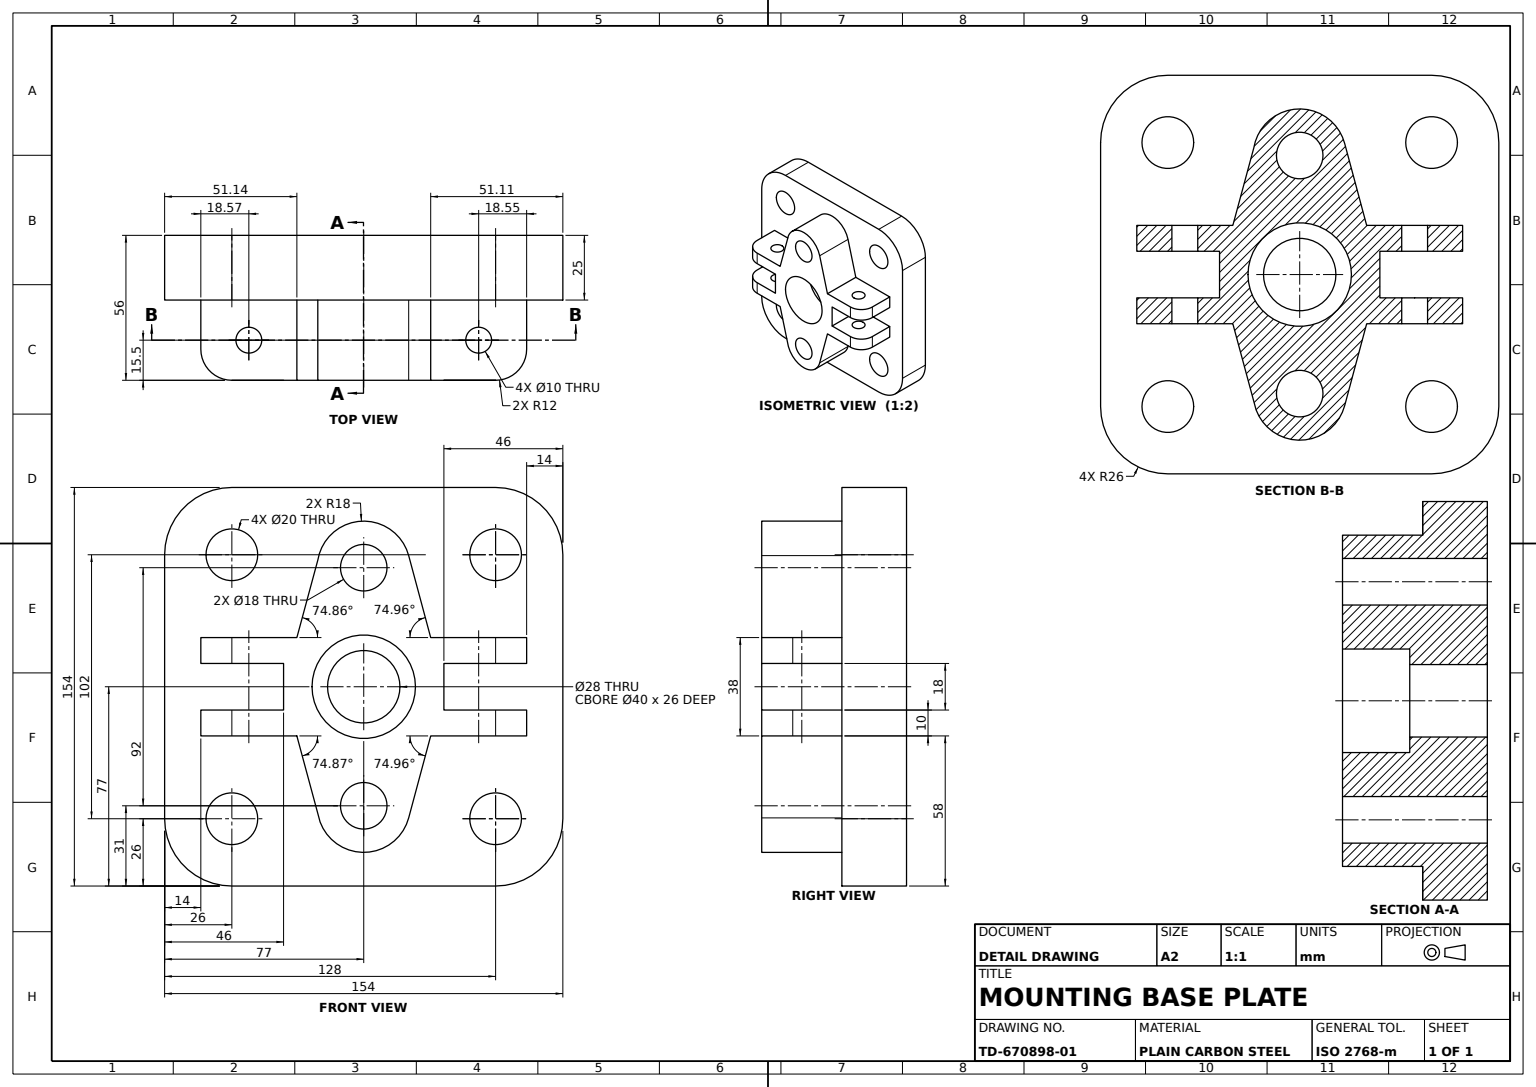
solid
v1 (97,77,56)
v2 (57,77,56)
e1 v1 v2 CIRCLE(AX(P(77,77,56),D(0,0,1),D(1,0,0)),20)
e2 v2 v1 CIRCLE(AX(P(77,77,56),D(0,0,1),D(1,0,0)),20)
v3 (86,31,56)
v4 (68,31,56)
e3 v3 v4 CIRCLE(AX(P(77,31,56),D(0,0,1),D(1,0,0)),9)
e4 v4 v3 CIRCLE(AX(P(77,31,56),D(0,0,1),D(1,0,0)),9)
v5 (108,86,56)
v6 (108,68,56)
e5 v5 v6 LINE
v7 (128,86,56)
e6 v5 v7 LINE
v8 (128,96,56)
e7 v7 v8 LINE
v9 (102.894203,96,56)
e8 v8 v9 LINE
v10 (94.383284,127.671343,56)
e9 v9 v10 LINE
v11 (59.235235,125.900538,56)
e10 v10 v11 CIRCLE(AX(P(77,123,56),D(0,0,1),D(1,0,0)),18)
v12 (51.142468,96,56)
e11 v12 v11 LINE
v13 (26,96,56)
e12 v13 v12 LINE
v14 (26,86,56)
e13 v13 v14 LINE
v15 (46,86,56)
e14 v15 v14 LINE
v16 (46,68,56)
e15 v16 v15 LINE
v17 (26,68,56)
e16 v16 v17 LINE
v18 (26,58,56)
e17 v17 v18 LINE
v19 (51.135796,58,56)
e18 v18 v19 LINE
v20 (60.132879,24.715079,56)
e19 v19 v20 LINE
v21 (94.383284,26.328657,56)
e20 v20 v21 CIRCLE(AX(P(77,31,56),D(0,0,1),D(1,0,0)),18)
v22 (102.894203,58,56)
e21 v22 v21 LINE
v23 (128,58,56)
e22 v23 v22 LINE
v24 (128,68,56)
e23 v23 v24 LINE
e24 v6 v24 LINE
v25 (68,123,56)
v26 (86,123,56)
e25 v25 v26 CIRCLE(AX(P(77,123,56),D(0,0,1),D(1,0,0)),9)
e26 v26 v25 CIRCLE(AX(P(77,123,56),D(0,0,1),D(1,0,0)),9)
face PLANE(AX(P(0,0,56),D(0,0,1),D(1,0,0))) [-e1 -e2] [-e3 -e4] [-e5 e6 e7 e8 e9 e10 -e11 -e12 e13 -e14 -e15 e16 e17 e18 e19 e20 -e21 -e22 e23 -e24] [-e25 -e26]
v27 (121.447101,68,35.5)
v28 (121.447101,58,35.5)
e27 v27 v28 LINE
v29 (121.447101,58,45.5)
e28 v28 v29 CIRCLE(AX(P(121.447101,58,40.5),D(0,-1,0),D(0,0,-1)),5)
v30 (121.447101,68,45.5)
e29 v30 v29 LINE
e30 v30 v27 CIRCLE(AX(P(121.447101,68,40.5),D(0,1,0),D(0,0,1)),5)
face CYL(AX(P(121.447101,154,40.5),D(0,-1,0),D(0,0,-1)),5) rev [e27 e28 -e29 e30]
v31 (68,123,0)
e31 v31 v25 LINE
v32 (86,123,0)
e32 v32 v31 CIRCLE(AX(P(77,123,0),D(0,0,1),D(1,0,0)),9)
e33 v32 v26 LINE
face CYL(AX(P(77,123,56),D(0,0,1),D(1,0,0)),9) rev [e26 -e31 -e32 e33]
v33 (91,77,0)
v34 (91,77,30)
e34 v33 v34 LINE
v35 (63,77,30)
e35 v35 v34 CIRCLE(AX(P(77,77,30),D(0,0,-1),D(1,0,0)),14)
v36 (63,77,0)
e36 v36 v35 LINE
e37 v33 v36 CIRCLE(AX(P(77,77,0),D(0,0,1),D(1,0,0)),14)
face CYL(AX(P(77,77,0),D(0,0,1),D(1,0,0)),14) rev [e34 -e35 -e36 -e37]
v37 (121.447101,96,45.5)
v38 (121.447101,86,45.5)
e38 v37 v38 LINE
v39 (121.447101,86,35.5)
e39 v39 v38 CIRCLE(AX(P(121.447101,86,40.5),D(0,1,0),D(0,0,1)),5)
v40 (121.447101,96,35.5)
e40 v40 v39 LINE
e41 v37 v40 CIRCLE(AX(P(121.447101,96,40.5),D(0,-1,0),D(1,0,0)),5)
face CYL(AX(P(121.447101,154,40.5),D(0,-1,0),D(0,0,-1)),5) rev [e38 -e39 -e40 -e41]
v41 (138,26,0)
v42 (118,26,0)
e42 v41 v42 CIRCLE(AX(P(128,26,0),D(0,0,1),D(1,0,0)),10)
e43 v42 v41 CIRCLE(AX(P(128,26,0),D(0,0,1),D(1,0,0)),10)
v43 (36,128,0)
v44 (16,128,0)
e44 v43 v44 CIRCLE(AX(P(26,128,0),D(0,0,1),D(1,0,0)),10)
e45 v44 v43 CIRCLE(AX(P(26,128,0),D(0,0,1),D(1,0,0)),10)
e46 v36 v33 CIRCLE(AX(P(77,77,0),D(0,0,1),D(1,0,0)),14)
v45 (138,128,0)
v46 (118,128,0)
e47 v45 v46 CIRCLE(AX(P(128,128,0),D(0,0,1),D(1,0,0)),10)
e48 v46 v45 CIRCLE(AX(P(128,128,0),D(0,0,1),D(1,0,0)),10)
e49 v31 v32 CIRCLE(AX(P(77,123,0),D(0,0,1),D(1,0,0)),9)
v47 (154,26,0)
v48 (154,128,0)
e50 v47 v48 LINE
v49 (128,0,0)
e51 v47 v49 CIRCLE(AX(P(128,26,0),D(0,0,-1),D(1,0,0)),26)
v50 (26,0,0)
e52 v50 v49 LINE
v51 (0,26,0)
e53 v50 v51 CIRCLE(AX(P(26,26,0),D(0,0,-1),D(1,0,0)),26)
v52 (0,128,0)
e54 v52 v51 LINE
v53 (26,154,0)
e55 v52 v53 CIRCLE(AX(P(26,128,0),D(0,0,-1),D(1,0,0)),26)
v54 (128,154,0)
e56 v54 v53 LINE
e57 v54 v48 CIRCLE(AX(P(128,128,0),D(0,0,-1),D(1,0,0)),26)
v55 (16,26,0)
v56 (36,26,0)
e58 v55 v56 CIRCLE(AX(P(26,26,0),D(0,0,1),D(1,0,0)),10)
e59 v56 v55 CIRCLE(AX(P(26,26,0),D(0,0,1),D(1,0,0)),10)
v57 (86,31,0)
v58 (68,31,0)
e60 v57 v58 CIRCLE(AX(P(77,31,0),D(0,0,1),D(1,0,0)),9)
e61 v58 v57 CIRCLE(AX(P(77,31,0),D(0,0,1),D(1,0,0)),9)
face PLANE(AX(P(0,0,0),D(0,0,1),D(1,0,0))) rev [e42 e43] [e44 e45] [e46 e37] [e47 e48] [e32 e49] [-e50 e51 -e52 e53 -e54 e55 -e56 e57] [e58 e59] [e60 e61]
v59 (16,128,25)
v60 (36,128,25)
e62 v59 v60 CIRCLE(AX(P(26,128,25),D(0,0,1),D(1,0,0)),10)
e63 v43 v60 LINE
e64 v44 v59 LINE
face CYL(AX(P(26,128,0),D(0,0,1),D(1,0,0)),10) rev [e62 -e63 -e45 e64]
e65 v40 v37 CIRCLE(AX(P(121.447101,96,40.5),D(0,-1,0),D(1,0,0)),5)
e66 v38 v39 CIRCLE(AX(P(121.447101,86,40.5),D(0,1,0),D(0,0,1)),5)
face CYL(AX(P(121.447101,154,40.5),D(0,-1,0),D(0,0,-1)),5) rev [-e38 -e65 e40 -e66]
v61 (26,154,25)
e67 v53 v61 LINE
v62 (128,154,25)
e68 v62 v61 LINE
e69 v62 v54 LINE
face PLANE(AX(P(154,154,25),D(0,-1,0),D(0,0,-1))) rev [e67 -e68 e69 e56]
v63 (32.567898,68,35.5)
v64 (32.567898,68,45.5)
e70 v63 v64 CIRCLE(AX(P(32.567898,68,40.5),D(0,-1,0),D(0,0,-1)),5)
e71 v64 v63 CIRCLE(AX(P(32.567898,68,40.5),D(0,-1,0),D(0,0,-1)),5)
v65 (14,68,44)
e72 v65 v17 CIRCLE(AX(P(26,68,44),D(0,1,0),D(0,0,-1)),12)
v66 (46,68,25)
e73 v16 v66 LINE
v67 (14,68,25)
e74 v66 v67 LINE
e75 v65 v67 LINE
face PLANE(AX(P(0,68,56),D(0,-1,0),D(0,0,-1))) rev [e70 e71] [e72 -e16 e73 e74 -e75]
e76 v60 v59 CIRCLE(AX(P(26,128,25),D(0,0,1),D(1,0,0)),10)
face CYL(AX(P(26,128,0),D(0,0,1),D(1,0,0)),10) rev [e63 e76 -e64 -e44]
v68 (32.567898,86,45.5)
v69 (32.567898,86,35.5)
e77 v68 v69 CIRCLE(AX(P(32.567898,86,40.5),D(0,-1,0),D(0,0,-1)),5)
e78 v69 v68 CIRCLE(AX(P(32.567898,86,40.5),D(0,-1,0),D(0,0,-1)),5)
v70 (14,86,44)
v71 (14,86,25)
e79 v70 v71 LINE
v72 (46,86,25)
e80 v72 v71 LINE
e81 v15 v72 LINE
e82 v14 v70 CIRCLE(AX(P(26,86,44),D(0,-1,0),D(0,0,-1)),12)
face PLANE(AX(P(0,86,56),D(0,-1,0),D(0,0,-1))) [-e77 -e78] [e79 -e80 -e81 e14 e82]
v73 (16,26,25)
v74 (36,26,25)
e83 v73 v74 CIRCLE(AX(P(26,26,25),D(0,0,1),D(1,0,0)),10)
e84 v56 v74 LINE
e85 v55 v73 LINE
face CYL(AX(P(26,26,0),D(0,0,1),D(1,0,0)),10) rev [e83 -e84 -e58 e85]
v75 (102.894203,96,25)
e86 v9 v75 LINE
v76 (94.383284,127.671343,25)
e87 v75 v76 LINE
e88 v10 v76 LINE
face PLANE(AX(P(120.024496,32.253724,56),D(-0.965737982,-0.259519075,0),D(0.259519075,-0.965737982,0))) rev [e86 e87 -e88 -e9]
e89 v57 v3 LINE
e90 v58 v4 LINE
face CYL(AX(P(77,31,56),D(0,0,1),D(1,0,0)),9) rev [-e60 e89 e3 -e90]
v77 (140,96,44)
e91 v8 v77 CIRCLE(AX(P(128,96,44),D(0,1,0),D(1,0,0)),12)
v78 (140,96,25)
e92 v77 v78 LINE
e93 v78 v75 LINE
face PLANE(AX(P(0,96,56),D(0,-1,0),D(1,0,0))) rev [e65 e41] [-e8 e91 e92 e93 -e86]
v79 (138,128,25)
v80 (118,128,25)
e94 v79 v80 CIRCLE(AX(P(128,128,25),D(0,0,1),D(1,0,0)),10)
e95 v46 v80 LINE
e96 v45 v79 LINE
face CYL(AX(P(128,128,0),D(0,0,1),D(1,0,0)),10) rev [e94 -e95 -e47 e96]
v81 (60.132879,24.715079,25)
e97 v20 v81 LINE
v82 (94.383284,26.328657,25)
e98 v81 v82 CIRCLE(AX(P(77,31,25),D(0,0,1),D(1,0,0)),18)
e99 v21 v82 LINE
face CYL(AX(P(77,31,56),D(0,0,-1),D(-1,0,0)),18) [e97 e98 -e99 -e20]
e100 v80 v79 CIRCLE(AX(P(128,128,25),D(0,0,1),D(1,0,0)),10)
face CYL(AX(P(128,128,0),D(0,0,1),D(1,0,0)),10) rev [-e48 e95 e100 -e96]
v83 (14,96,44)
e101 v83 v13 CIRCLE(AX(P(26,96,44),D(0,1,0),D(0,0,1)),12)
e102 v70 v83 LINE
face CYL(AX(P(26,0,44),D(0,1,0),D(0,0,1)),12) [-e82 -e13 -e101 -e102]
v84 (51.135796,58,25)
e103 v19 v84 LINE
e104 v84 v81 LINE
face PLANE(AX(P(62.264169,16.83032,56),D(0.965354932,0.26094033,0),D(-0.26094033,0.965354932,0))) rev [-e19 e103 e104 -e97]
v85 (154,26,25)
e105 v85 v47 LINE
v86 (128,0,25)
e106 v86 v85 CIRCLE(AX(P(128,26,25),D(0,0,1),D(1,0,0)),26)
e107 v49 v86 LINE
face CYL(AX(P(128,26,25),D(0,0,-1),D(-1,0,0)),26) [-e105 -e106 -e107 -e51]
v87 (0,128,25)
e108 v87 v52 LINE
e109 v61 v87 CIRCLE(AX(P(26,128,25),D(0,0,1),D(1,0,0)),26)
face CYL(AX(P(26,128,25),D(0,0,-1),D(-1,0,0)),26) [-e55 -e108 -e109 -e67]
v88 (57,77,30)
v89 (97,77,30)
e110 v88 v89 CIRCLE(AX(P(77,77,30),D(0,0,1),D(1,0,0)),20)
e111 v88 v2 LINE
e112 v89 v1 LINE
face CYL(AX(P(77,77,30),D(0,0,1),D(1,0,0)),20) rev [-e110 e111 e2 -e112]
e113 v74 v73 CIRCLE(AX(P(26,26,25),D(0,0,1),D(1,0,0)),10)
face CYL(AX(P(26,26,0),D(0,0,1),D(1,0,0)),10) rev [-e85 -e59 e84 e113]
v90 (0,26,25)
e114 v51 v90 LINE
e115 v87 v90 LINE
face PLANE(AX(P(0,154,25),D(1,0,0),D(0,0,-1))) rev [e54 e114 -e115 e108]
v91 (14,58,44)
e116 v18 v91 CIRCLE(AX(P(26,58,44),D(0,-1,0),D(0,0,1)),12)
e117 v91 v65 LINE
face CYL(AX(P(26,0,44),D(0,1,0),D(0,0,1)),12) [-e116 -e17 -e72 -e117]
v92 (14,96,25)
e118 v83 v92 LINE
e119 v71 v92 LINE
face PLANE(AX(P(14,0,56),D(-1,0,0),D(0,0,1))) [e102 e118 -e119 -e79]
e120 v34 v35 CIRCLE(AX(P(77,77,30),D(0,0,-1),D(1,0,0)),14)
face CYL(AX(P(77,77,0),D(0,0,1),D(1,0,0)),14) rev [e36 -e120 -e34 -e46]
e121 v89 v88 CIRCLE(AX(P(77,77,30),D(0,0,1),D(1,0,0)),20)
face PLANE(AX(P(77,77,30),D(0,0,1),D(1,0,0))) [e121 e110] [e120 e35]
e122 v66 v72 LINE
face PLANE(AX(P(46,0,56),D(-1,0,0),D(0,-1,0))) [-e73 e15 e81 -e122]
v93 (51.142468,96,25)
v94 (59.235235,125.900538,25)
e123 v93 v94 LINE
e124 v12 v93 LINE
e125 v11 v94 LINE
face PLANE(AX(P(23.442216,-6.344782,56),D(-0.965269496,0.261256196,0),D(-0.261256196,-0.965269496,0))) [-e123 -e124 e11 e125]
e126 v27 v30 CIRCLE(AX(P(121.447101,68,40.5),D(0,1,0),D(0,0,1)),5)
e127 v29 v28 CIRCLE(AX(P(121.447101,58,40.5),D(0,-1,0),D(0,0,-1)),5)
face CYL(AX(P(121.447101,154,40.5),D(0,-1,0),D(0,0,-1)),5) rev [-e27 e126 e29 e127]
v95 (26,0,25)
e128 v90 v95 CIRCLE(AX(P(26,26,25),D(0,0,1),D(1,0,0)),26)
e129 v95 v50 LINE
face CYL(AX(P(26,26,25),D(0,0,-1),D(-1,0,0)),26) [-e128 -e114 -e53 -e129]
e130 v76 v94 CIRCLE(AX(P(77,123,25),D(0,0,1),D(1,0,0)),18)
face CYL(AX(P(77,123,56),D(0,0,-1),D(-1,0,0)),18) [e88 e130 -e125 -e10]
e131 v95 v86 LINE
face PLANE(AX(P(0,0,25),D(0,1,0),D(0,0,1))) rev [e52 e107 -e131 e129]
v96 (108,86,25)
e132 v5 v96 LINE
v97 (108,68,25)
e133 v6 v97 LINE
e134 v96 v97 LINE
face PLANE(AX(P(108,0,56),D(1,0,0),D(0,0,-1))) [-e132 e5 e133 -e134]
v98 (14,58,25)
e135 v91 v98 LINE
e136 v98 v84 LINE
v99 (32.567898,58,35.5)
v100 (32.567898,58,45.5)
e137 v99 v100 CIRCLE(AX(P(32.567898,58,40.5),D(0,-1,0),D(0,0,-1)),5)
e138 v100 v99 CIRCLE(AX(P(32.567898,58,40.5),D(0,-1,0),D(0,0,-1)),5)
face PLANE(AX(P(0,58,56),D(0,1,0),D(0,0,1))) rev [e135 e136 -e103 -e18 e116] [-e137 -e138]
e139 v64 v100 LINE
e140 v63 v99 LINE
face CYL(AX(P(32.567898,154,40.5),D(0,-1,0),D(0,0,-1)),5) rev [-e71 e139 e138 -e140]
v101 (32.567898,96,35.5)
v102 (32.567898,96,45.5)
e141 v101 v102 CIRCLE(AX(P(32.567898,96,40.5),D(0,1,0),D(0,0,1)),5)
e142 v102 v101 CIRCLE(AX(P(32.567898,96,40.5),D(0,1,0),D(0,0,1)),5)
e143 v92 v93 LINE
face PLANE(AX(P(0,96,56),D(0,1,0),D(0,0,1))) [-e141 -e142] [e101 e12 e124 -e143 -e118]
face CYL(AX(P(77,31,56),D(0,0,1),D(1,0,0)),9) rev [-e61 e90 e4 -e89]
e144 v102 v68 LINE
e145 v101 v69 LINE
face CYL(AX(P(32.567898,154,40.5),D(0,-1,0),D(0,0,-1)),5) rev [e144 e77 -e145 e141]
e146 v67 v98 LINE
face PLANE(AX(P(14,0,56),D(1,0,0),D(0,0,-1))) rev [e146 -e135 e117 e75]
v103 (140,86,44)
v104 (140,86,25)
e147 v103 v104 LINE
e148 v103 v7 CIRCLE(AX(P(128,86,44),D(0,-1,0),D(0,0,1)),12)
e149 v96 v104 LINE
face PLANE(AX(P(0,86,56),D(0,1,0),D(0,0,1))) rev [-e147 e148 -e6 e132 e149] [e66 e39]
v105 (102.894203,58,25)
e150 v105 v82 LINE
e151 v22 v105 LINE
face PLANE(AX(P(81.427872,-21.881801,56),D(0.965737982,-0.259519075,0),D(0.259519075,0.965737982,0))) [-e150 -e151 e21 e99]
e152 v104 v78 LINE
e153 v77 v103 LINE
face PLANE(AX(P(140,0,56),D(-1,0,0),D(0,0,1))) rev [e147 e152 -e92 e153]
face CYL(AX(P(32.567898,154,40.5),D(0,-1,0),D(0,0,-1)),5) rev [e78 -e144 e142 e145]
v106 (140,58,25)
e154 v106 v105 LINE
v107 (140,58,44)
e155 v107 v106 LINE
e156 v107 v23 CIRCLE(AX(P(128,58,44),D(0,-1,0),D(0,0,-1)),12)
face PLANE(AX(P(0,58,56),D(0,-1,0),D(0,0,-1))) [e151 -e154 -e155 e156 e22] [-e28 -e127]
face CYL(AX(P(128,0,44),D(0,-1,0),D(0,0,-1)),12) [-e148 -e153 -e91 -e7]
v108 (154,128,25)
e157 v108 v62 CIRCLE(AX(P(128,128,25),D(0,0,1),D(1,0,0)),26)
e158 v48 v108 LINE
face CYL(AX(P(128,128,25),D(0,0,-1),D(-1,0,0)),26) [-e57 -e69 -e157 -e158]
v109 (118,26,25)
e159 v42 v109 LINE
v110 (138,26,25)
e160 v109 v110 CIRCLE(AX(P(128,26,25),D(0,0,1),D(1,0,0)),10)
e161 v41 v110 LINE
face CYL(AX(P(128,26,0),D(0,0,1),D(1,0,0)),10) rev [e159 e160 -e161 -e43]
v111 (140,68,44)
v112 (140,68,25)
e162 v111 v112 LINE
e163 v97 v112 LINE
e164 v24 v111 CIRCLE(AX(P(128,68,44),D(0,1,0),D(0,0,1)),12)
face PLANE(AX(P(0,68,56),D(0,1,0),D(0,0,1))) [e162 -e163 -e133 e24 e164] [-e30 -e126]
face CYL(AX(P(77,77,30),D(0,0,1),D(1,0,0)),20) rev [-e111 -e121 e112 e1]
e165 v110 v109 CIRCLE(AX(P(128,26,25),D(0,0,1),D(1,0,0)),10)
face CYL(AX(P(128,26,0),D(0,0,1),D(1,0,0)),10) rev [e161 e165 -e159 -e42]
face CYL(AX(P(77,123,56),D(0,0,1),D(1,0,0)),9) rev [-e33 -e49 e31 e25]
e166 v111 v107 LINE
e167 v112 v106 LINE
face PLANE(AX(P(140,0,56),D(1,0,0),D(0,0,-1))) [-e162 e166 e155 -e167]
face CYL(AX(P(128,0,44),D(0,-1,0),D(0,0,-1)),12) [-e166 -e164 -e23 -e156]
e168 v85 v108 LINE
face PLANE(AX(P(0,0,25),D(0,0,1),D(1,0,0))) [-e100 -e94] [e122 e80 e119 e143 e123 -e130 -e87 -e93 -e152 -e149 e134 e163 e167 e154 e150 -e98 -e104 -e136 -e146 -e74] [-e76 -e62] [-e160 -e165] [e109 e115 e128 e131 e106 e168 e157 e68] [-e83 -e113]
face CYL(AX(P(32.567898,154,40.5),D(0,-1,0),D(0,0,-1)),5) rev [e137 -e139 -e70 e140]
face PLANE(AX(P(154,0,25),D(-1,0,0),D(0,0,1))) rev [e105 e50 e158 -e168]
